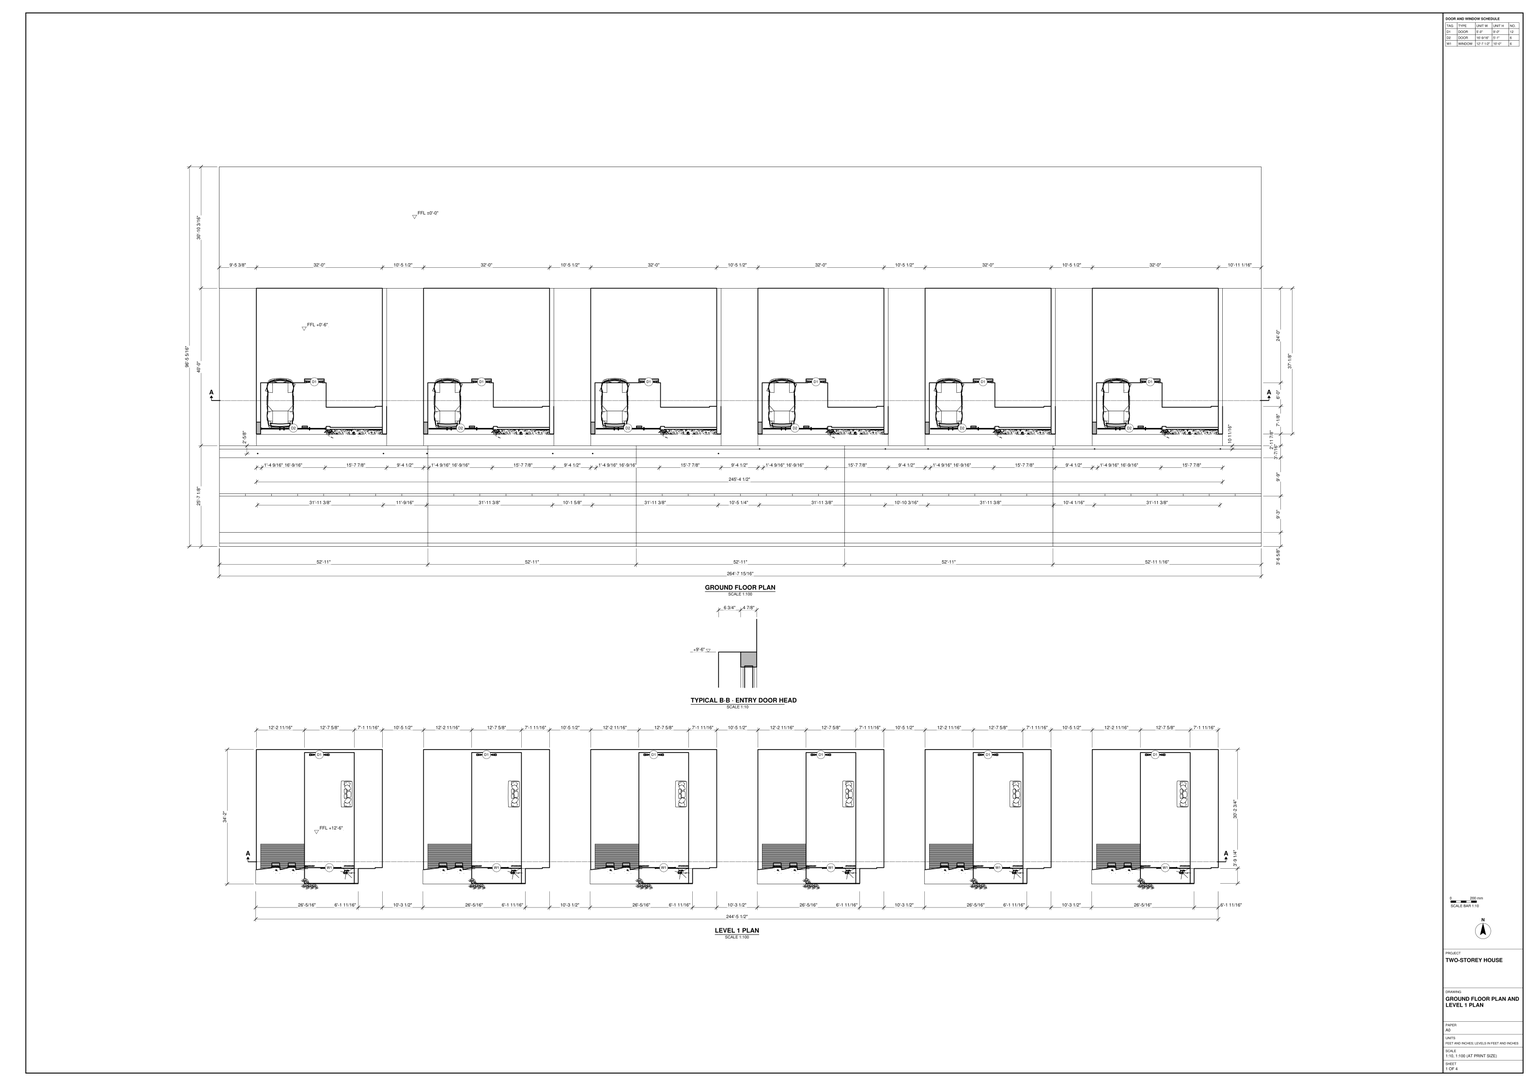
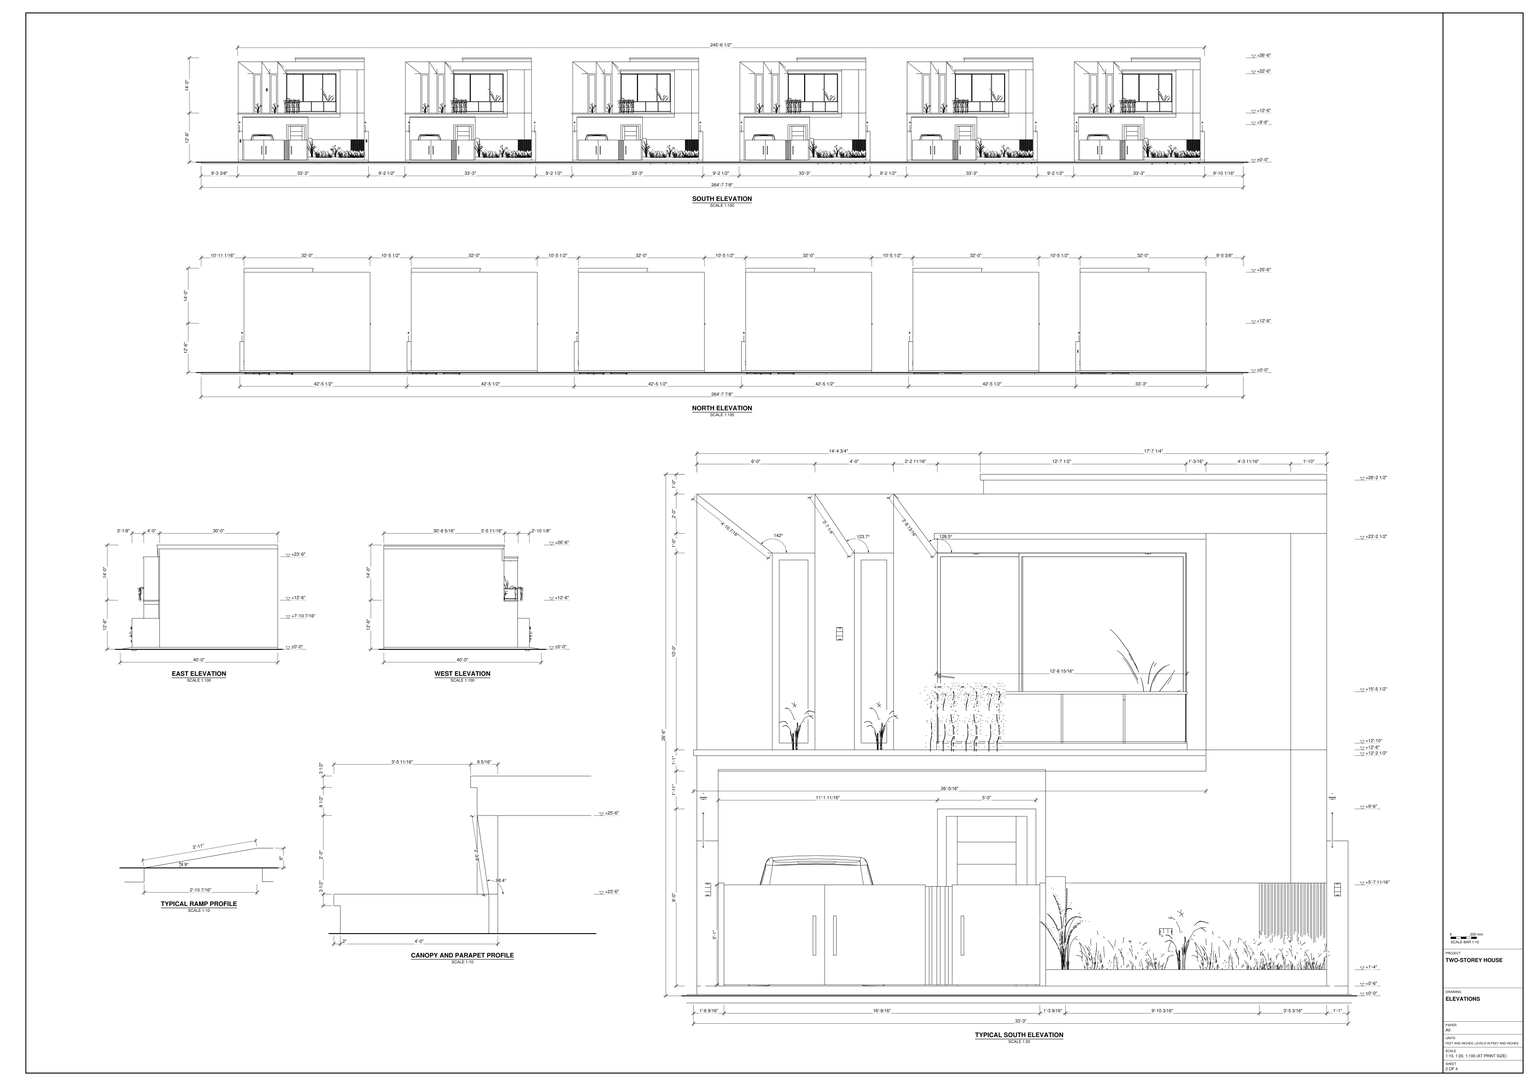
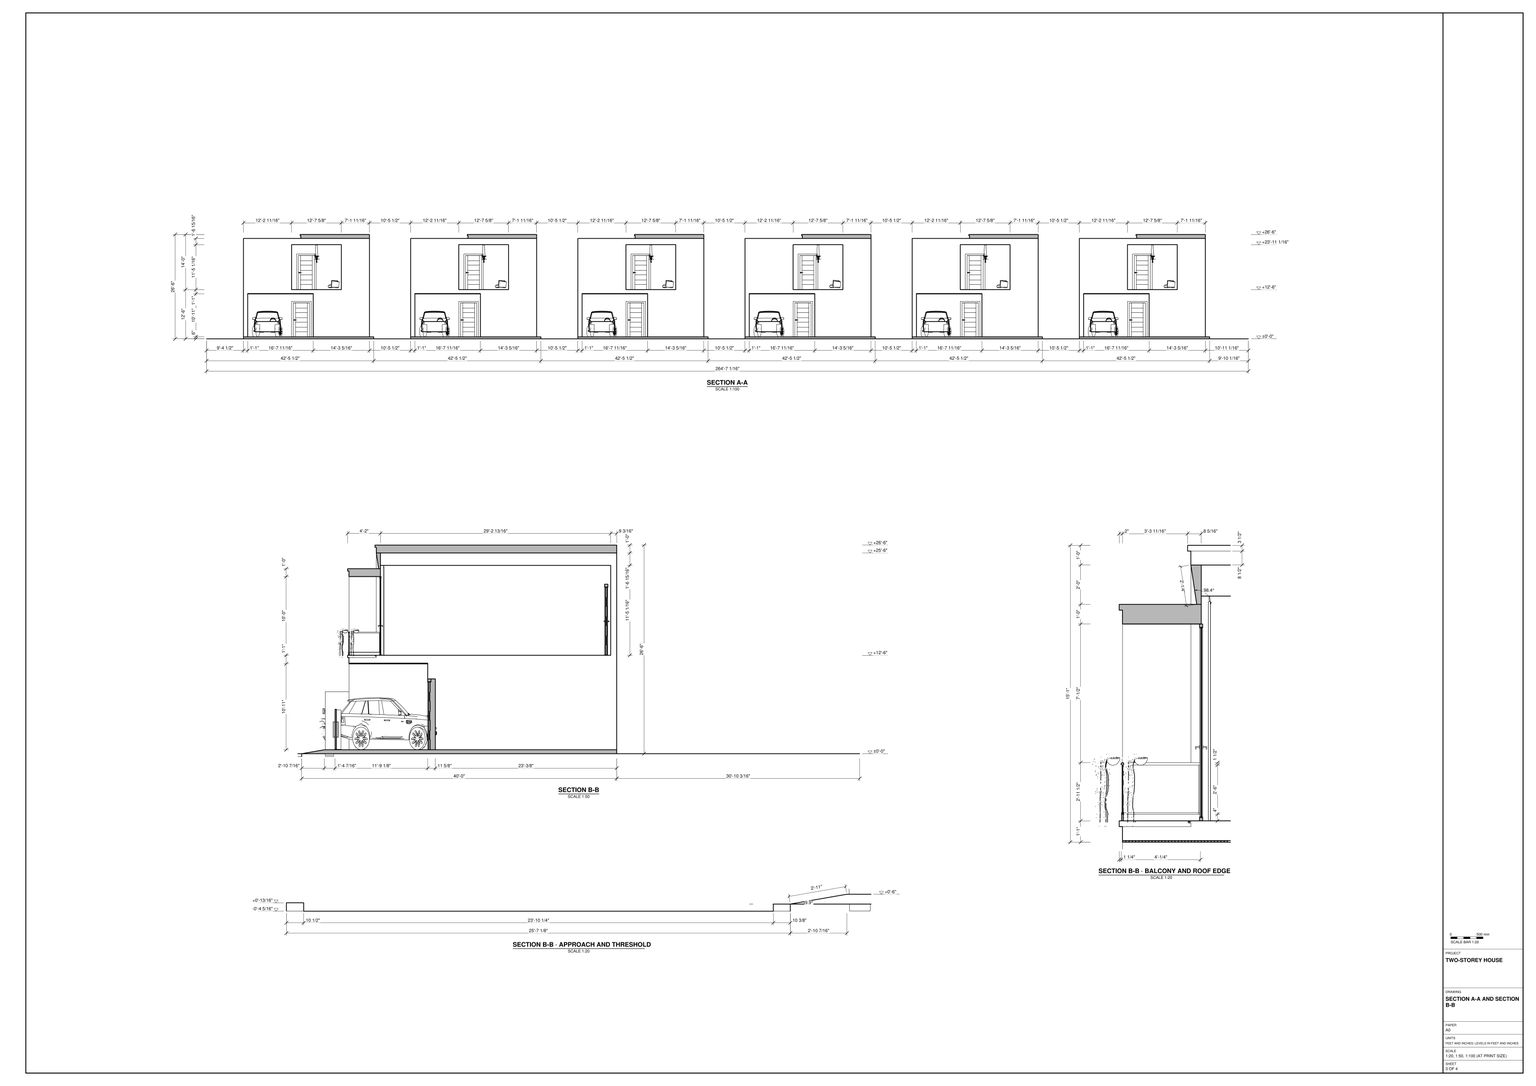
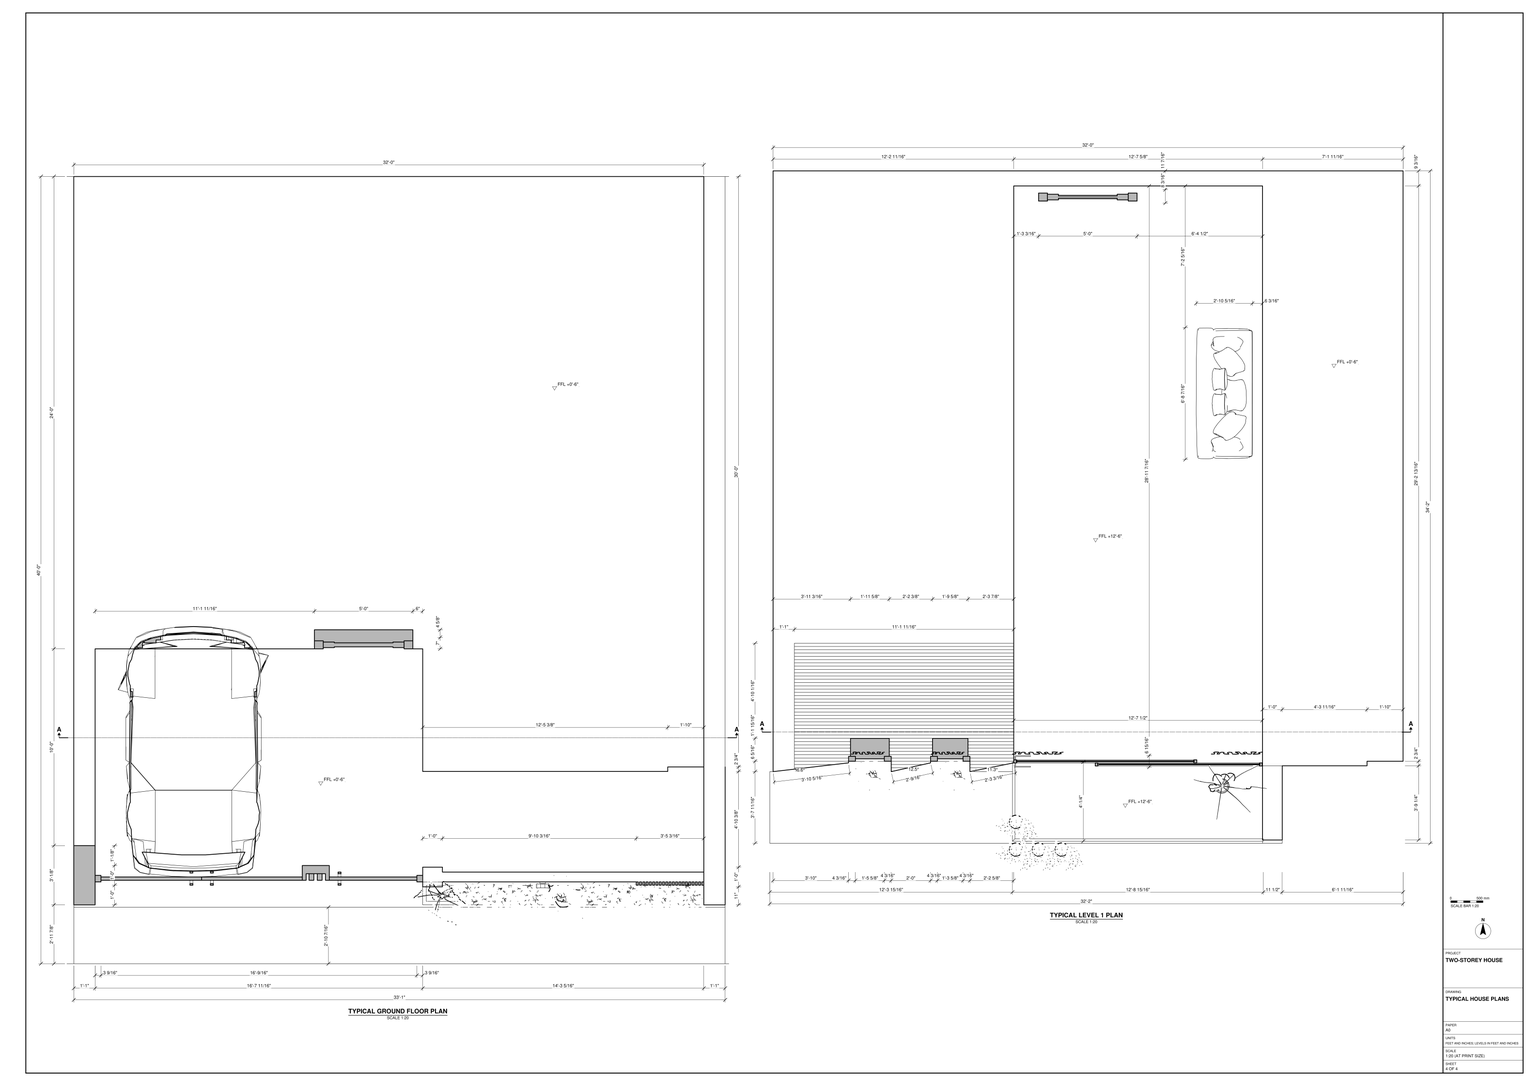
Build the six houses and their shared site in SketchUp from task_files/diagram_01.pdf. Work in feet and inches. The overall model extents are 264'-7 15/16" along the row, 96'-5 5/16" from front to back and 26'-10 5/16" in height. Set the ground-floor datum at ±0'-0" and the upper floor at +12'-6".

Use the ground-floor plan to set out the site edges, the approach across the south frontage and the gaps between houses. Model the walls at the thicknesses drawn, with floor slabs, door and window openings, flat roofs and parapets. At each frontage, form the ramped threshold, gate, covered parking bay and recessed entry. Above the bay, model the projecting balcony slab, front guard, tall fins and framed window. Use the sections to distinguish the canopy over the balcony from the higher roof edge. Include the upper-floor seating at the size and position shown in plan, together with the parked cars and planting shown in elevation. Cars, plants and other loose items may be any suitable library components.

Keep shell elements such as walls, slabs and roofs, and each furniture or joinery piece, in separate groups or components. Use components for repeated parts. Save one SketchUp model as output_files/row_of_six_two_storey_houses.skp.

# SketchUp Ruby script. Lengths in inches.
U = 1.inch
M = Sketchup.active_model
def pt(a) = Geom::Point3d.new(a.map { |v| v * U })
def face(e, loops, mat)
  f = e.add_face(loops[0].map { |a| pt(a) })
  loops[1..].each { |l| e.add_face(l.map { |a| pt(a) }).erase! }
  f.material = f.back_material = mat if mat
  f
end
# faces: each face lists its corners as indices into pts; further lists are holes
def faces(e, pts, list, mat = nil) = list.each { |f| face(e, (f[0].is_a?(Array) ? f : [f]).map { |l| l.map { |i| pts[i] } }, mat) }
# xy, xz, yz: faces in a plane at the given z, y or x. An outline is a flat list of corners, or four numbers for a rectangle; further outlines are holes
def ring(l) = l.size == 4 ? [[l[0], l[1]], [l[2], l[1]], [l[2], l[3]], [l[0], l[3]]] : l.each_slice(2).to_a
def flat(e, list, mat, &to3) = list.each { |f| face(e, (f[0].is_a?(Array) ? f : [f]).map { |l| ring(l).map { |u, v| to3.(u, v) } }, mat) }
def xy(e, z, list, mat = nil) = flat(e, list, mat) { |x, y| [x, y, z] }
def xz(e, y, list, mat = nil) = flat(e, list, mat) { |x, z| [x, y, z] }
def yz(e, x, list, mat = nil) = flat(e, list, mat) { |y, z| [x, y, z] }
def lines(e, pts, list) = list.each { |a, b| e.add_line(pt(pts[a]), pt(pts[b])) }
# prism: a flat outline (further loops are holes) pulled along v
def prism(e, loops, v, mat = nil)
  f = face(e, loops, mat); d = Geom::Vector3d.new(v.map { |x| x * U })
  f.pushpull(f.normal.samedirection?(d) ? d.length : -d.length)
end
def box(e, o, s, mat = nil) = prism(e, [[o, [o[0] + s[0], o[1], o[2]], [o[0] + s[0], o[1] + s[1], o[2]], [o[0], o[1] + s[1], o[2]]]], [0, 0, s[2]], mat)
def at(x, y, z, deg = 0) = Geom::Transformation.translation(pt([x, y, z])) * Geom::Transformation.rotation(ORIGIN, Z_AXIS, deg.degrees)
def axes(o, x, y, z) = Geom::Transformation.new([*x, 0, *y, 0, *z, 0, *pt(o).to_a, 1])
def part(name) = M.definitions.add(name)
# library, detail: a bought-in or finely detailed component or shape, given as its bounding box
def library(name, o, s) = part(name).tap { |d| box(d.entities, o, s) }
def detail(e, o, s) = box(e.add_group.entities, o, s)
def put(e, d, t, mat = nil) = e.add_instance(d, t).tap { |i| i.material = mat if mat }
def group(e, t, mat = nil) = e.add_group.tap { |g| g.transformation = t; g.material = mat if mat }.entities
root = M.entities
M.materials.add("Aluminum_Anodized_DarkGray").color = [72, 73, 74]
M.materials.add("[Asphalt_New]1").color = [67, 60, 62]
M.materials.add("[Color M09]").color = [0, 0, 0]
M.materials.add("[Color_000]").color = [255, 255, 255]
M.materials.add("[Grass Dark Green]").color = [106, 157, 55]
M.materials.add("[Pavers with Grass Brick]").color = [187, 192, 176]
M.materials.add("[Stone_Masonry_Multi]").color = [182, 175, 164]
M.materials.add("[Translucent Glass Gray]").color = [128, 128, 128]
M.materials["[Translucent Glass Gray]"].alpha = 0.5
M.materials.add("[Wood Veneer 01]").color = [120, 70, 37]
M.materials.add("polished steel").color = [183, 187, 190]
M.materials.add("polished_ Blacktop Old 01").color = [132, 136, 139]
M.materials.add("steel").color = [179, 179, 179]
c1 = library("Sliding windows",[297.42,-0.89,0.35],[192.38,8.85,122.84])
c2 = library("Pendente Fluire_RE005 ø28x74cm",[-3.08,-3.22,-55.33],[13.79,12.06,55.33])
c3 = part("faewg")
xy(c3.entities,0,[[0,-3,2,0]])
xy(c3.entities,1,[[0,-2,2,0]])
xy(c3.entities,23,[[0,-2,2,0]])
xy(c3.entities,24,[[0,-3,2,0]])
xz(c3.entities,-3,[[0,0,2,24]],"polished steel")
xz(c3.entities,-2,[[0,1,2,23]])
xz(c3.entities,0,[[0,0,2,1],[0,23,2,24]])
yz(c3.entities,0,[[-3,0,-3,24,0,24,0,23,-2,23,-2,1,0,1,0,0]])
yz(c3.entities,2,[[-3,0,0,0,0,1,-2,1,-2,23,0,23,0,24,-3,24]])
c4 = part("e3f")
xy(c4.entities,0,[[0,-2,59.93,0]])
xy(c4.entities,18,[[51.93,-5,53.93,-2]],"steel")
xy(c4.entities,19,[[51.93,-4,53.93,-2]],"steel")
xy(c4.entities,41,[[51.93,-4,53.93,-2]],"steel")
xy(c4.entities,42,[[51.93,-5,53.93,-2]],"steel")
xy(c4.entities,61,[[0,-2,59.93,0]],"[Wood Veneer 01]")
xz(c4.entities,-5,[[51.93,18,53.93,42]],"[Color M09]")
xz(c4.entities,-4,[[51.93,19,53.93,41]],"steel")
xz(c4.entities,-2,[[[0,0,59.93,61],[51.93,41,53.93,42],[51.93,18,53.93,19]]],"[Wood Veneer 01]")
xz(c4.entities,-2,[[51.93,18,53.93,19],[51.93,41,53.93,42]],"steel")
xz(c4.entities,0,[[0,0,59.93,61]],"[Wood Veneer 01]")
yz(c4.entities,0,[[-2,0,0,61]])
yz(c4.entities,51.93,[[-5,18,-5,42,-2,42,-2,41,-4,41,-4,19,-2,19,-2,18]],"[Color M09]")
yz(c4.entities,53.93,[[-5,18,-2,18,-2,19,-4,19,-4,41,-2,41,-2,42,-5,42]],"[Color M09]")
yz(c4.entities,59.93,[[-2,0,0,61]])
put(c4.entities,c3,axes([51.93,0,42],[1,0,0],[0,-1,0],[0,0,-1]),"steel")
c5 = part("reg")
xy(c5.entities,0,[[-8.95,3,59.93,5]],"[Wood Veneer 01]")
xy(c5.entities,18,[[51.93,0,53.93,3]],"[Wood Veneer 01]")
xy(c5.entities,19,[[51.93,1,53.93,3]],"[Color M09]")
xy(c5.entities,41,[[51.93,1,53.93,3]],"[Color M09]")
xy(c5.entities,42,[[51.93,0,53.93,3]],"[Color M09]")
xy(c5.entities,61,[[-8.95,3,59.93,5]],"[Wood Veneer 01]")
xz(c5.entities,0,[[51.93,18,53.93,42]],"[Color M09]")
xz(c5.entities,1,[[51.93,19,53.93,41]],"[Wood Veneer 01]")
xz(c5.entities,3,[[[-8.95,0,59.93,61],[51.93,41,53.93,42],[51.93,18,53.93,19]],[51.93,18,53.93,19],[51.93,41,53.93,42]],"[Wood Veneer 01]")
xz(c5.entities,5,[[-8.95,0,59.93,61]],"[Wood Veneer 01]")
yz(c5.entities,-8.95,[[3,0,5,61]],"[Wood Veneer 01]")
yz(c5.entities,51.93,[[0,18,0,42,3,42,3,41,1,41,1,19,3,19,3,18]],"[Color M09]")
yz(c5.entities,53.93,[[0,18,3,18,3,19,1,19,1,41,3,41,3,42,0,42]],"[Color M09]")
yz(c5.entities,59.93,[[3,0,5,61]],"[Wood Veneer 01]")
put(c5.entities,c3,axes([51.93,5.4375,42],[1,0,0],[0,-1,0],[0,0,-1]),"steel")
c6 = part("main gate")
g1 = group(c6.entities,at(416.55,56.79,1))
put(g1,c4,at(0,5,0))
put(g1,c5,axes([207.23,0,0],[-1,0,0],[0,1,0],[0,0,1]),"[Grass Dark Green]")
put(g1,c5,at(87.36,0,0),"[Grass Dark Green]")
g2 = group(g1,at(59.93,12,0),"polished_ Blacktop Old 01")
prism(g2,[[[0,0,0],[18.48,0,0],[18.48,-9,0],[15.84,-9,0],[15.84,-5,0],[2.64,-5,0],[2.64,-9,0],[0,-9,0]]],[0,0,60],"[Color M09]")
g3 = group(g1,at(-173.38,3,0),"[Grass Dark Green]")
prism(g3,[[[241.55,4,0],[241.55,4,4],[241.55,4,56],[241.55,4,60],[241.55,0,60],[241.55,0,0]]],[-3.3,0,0])
prism(g3,[[[247.19,4,0],[247.19,4,4],[247.19,4,56],[247.19,4,60],[247.19,0,60],[247.19,0,0]]],[-3.3,0,0])
c7 = library("cay+chuoi",[26.89,19.66,0.52],[41.96,45.65,69.71])
c8 = library("Areca palm plant",[0,0,0],[49.1,36.6,54.46])
c9 = library("Land Rover Range Rover Sport",[-42.64,-96.16,0],[85.02,188.78,73.23])
c10 = library("TS_VASO+GANCHOS-PARA-PENDURAR\#1",[-17.61,-15.74,-70.29],[36.55,50.24,77.96])
c11 = library("Glass Railing\#1",[-152.43,-0.75,0],[152.93,48.27,35.5])
c12 = part("Group\#12")
box(c12.entities,[0,0,0],[3.5625,4,62.75])
c13 = library("Group\#13",[0,0,0],[171.32,12,66.75])
c14 = library("door by lz",[5.91,-4.92,0],[35.43,6.61,78.47])
c15 = part("Group\#61")
p = [[0,1.89,0.38],[0,1.89,1.61],[0,0.72,0],[0,0,0.99],[0,0.72,1.99]]
lines(c15.entities,p,[[0,1],[2,0],[3,2],[4,3],[1,4]])
c16 = part("Pleated curtain panel")
p = [[20.45,2.26,80],[20.78,2.41,80]]
lines(c16.entities,p,[[0,1]])
detail(c16.entities,[0,1.93,2.7],[20.05,3.87,77.3])
put(c16.entities,c15,at(9.77,5.02,80,-180))
put(c16.entities,c15,at(11.91,5.02,80,-180))
put(c16.entities,c15,at(13.54,5.02,80,-180))
put(c16.entities,c15,at(7.29,5.02,80,-180))
put(c16.entities,c15,at(6.18,5.02,80,-180))
put(c16.entities,c15,at(8.69,5.02,80,-180))
put(c16.entities,c15,at(17.42,5.04,80,-180))
put(c16.entities,c15,at(18.86,5.04,80,-180))
put(c16.entities,c15,at(15.09,5.02,80,-180))
put(c16.entities,c15,at(16.66,5.04,80,-180))
put(c16.entities,c15,at(2.54,5.02,80,-180))
put(c16.entities,c15,at(1.38,5.02,80,-180))
put(c16.entities,c15,at(4.1,5.02,80,-180))
c17 = library("sofaD71839)",[0.35,-39.08,0.31],[80.46,34.29,30.24])
c18 = library("Group211\#1",[-99.84,-60,0],[199.68,120,1])
c19 = library("Group275\#1",[-75.83,-24,0],[151.66,48,0.08])
c20 = part("Group")
xy(c20.entities,0,[[0,-36.125,13,0],[0,0,0,408,384,408,384,48,362.03,48,362.03,45.24,212.68,45.24,212.68,120,206.68,120,206.68,131.625,146.68,131.625,146.68,120,13,120,13,0]])
xy(c20.entities,108,[[146.68,120,206.68,131.625]])
xy(c20.entities,131,[[212.68,0,310.34,45.24]])
xy(c20.entities,140.5,[[-2,-2,310.34,0],[-2,0,0,41.6875]],"Aluminum_Anodized_DarkGray")
xy(c20.entities,144,[[-2,-2,298.34,-2,298.34,398.8125,146.6875,398.8125,146.6875,41.6875,120,41.6875,120,48,96,48,96,47.02,72,41.6875,72,48,46,48,46,47.02,0,41.6875,-2,41.6875],[298.34,-2,310.34,0],[120,41.6875,146.68,41.6875,146.68,47.02],[146.68,41.6875,146.6875,41.6875,146.6875,48,146.68,47.02]])
xy(c20.entities,144,[[46,48,72,51],[96,48,120,51]],"[Color M09]")
xy(c20.entities,148.1875,[[47.1875,51,70.8125,61.9375],[97.1875,51,118.8125,61.9375]])
xy(c20.entities,148.1875,[[50.1875,48,67.8125,49.5],[100.1875,48,115.8125,49.5],[50.1875,49.5,67.8125,51],[100.1875,49.5,115.8125,51]],"[Color M09]")
xy(c20.entities,259.8125,[[50.1875,48,67.8125,49.5],[100.1875,48,115.8125,49.5],[50.1875,49.5,67.8125,51],[100.1875,49.5,115.8125,51]],"[Color M09]")
xy(c20.entities,262.8125,[[47.1875,51,70.8125,61.9375],[97.1875,51,118.8125,61.9375]])
xy(c20.entities,264,[[146.68,41.6875,146.68,47.02,146.6875,48,146.6875,41.6875],[46,47.02,72,48],[96,47.02,120,48],[146.68,47.02,146.68,48,146.6875,48]])
xy(c20.entities,264,[[46,48,72,51],[96,48,120,51]],"[Color M09]")
xy(c20.entities,272.5,[[144.68,-2,310.34,0],[144.68,0,146.68,45.24]],"Aluminum_Anodized_DarkGray")
xy(c20.entities,276,[[144.68,-2,310.34,45.24],[146.68,45.24,310.34,48],[310.34,45.24,362.03,48],[362.03,45.24,384,48]])
xy(c20.entities,281.0625,[[146.6875,48,298.34,398.8125]])
xy(c20.entities,300,[[0,41.6875,120,41.6875,120,47.02,146.68,48,384,48,384,408,0,408],[120,41.6875,146.68,48,120,47.02],[120,41.6875,384,41.6875,384,48,146.68,48]])
xz(c20.entities,-2,[[-2,140.5,310.34,144],[144.68,272.5,310.34,276]],"Aluminum_Anodized_DarkGray")
xz(c20.entities,0,[[0,0,13,88.44]])
xz(c20.entities,0,[[0,88.44,13,88.44,13,131,310.34,131,310.34,140.5,0,140.5],[298.34,144,310.34,144,310.34,272.5,146.68,272.5,146.68,264,298.34,264]],"Aluminum_Anodized_DarkGray")
xz(c20.entities,41.6875,[[-2,140.5,0,144]])
xz(c20.entities,45.24,[[212.68,0,362.03,0,362.03,144,310.34,144,310.34,131,212.68,131],[310.34,144,362.03,276],[144.68,272.5,146.68,276]])
xz(c20.entities,47.02,[[0,264,46,264,0,300],[120,264,120,300,146.68,264]])
xz(c20.entities,48,[[362.03,0,384,144],[362.03,144,384,276],[146.68,264,146.6875,276],[146.6875,264,298.34,276],[146.68,276,146.6875,300],
  [146.6875,276,298.34,281.0625],[298.34,276,384,276,384,300,146.6875,300,146.6875,281.0625,298.34,281.0625]])
xz(c20.entities,48,[[[46,144,72,264],[50.1875,148.1875,67.8125,259.8125]],[[96,144,120,264],[100.1875,148.1875,115.8125,259.8125]]],"[Color M09]")
xz(c20.entities,49.5,[[50.1875,148.1875,67.8125,259.8125],[100.1875,148.1875,115.8125,259.8125]],"[Translucent Glass Gray]")
xz(c20.entities,51,[[47.1875,148.1875,50.1875,262.8125],[67.8125,148.1875,70.8125,262.8125],[97.1875,148.1875,100.1875,262.8125],[115.8125,148.1875,118.8125,262.8125],[50.1875,259.8125,67.8125,262.8125],
  [100.1875,259.8125,115.8125,262.8125]])
xz(c20.entities,51,[[[46,144,72,264],[47.1875,148.1875,70.8125,262.8125]],[[96,144,120,264],[97.1875,148.1875,118.8125,262.8125]]],"[Color M09]")
xz(c20.entities,61.9375,[[47.1875,148.1875,70.8125,262.8125],[97.1875,148.1875,118.8125,262.8125]])
xz(c20.entities,120,[[13,0,146.68,0,146.68,108,206.68,108,206.68,0,212.68,0,212.68,131,13,131]])
xz(c20.entities,131.625,[[146.68,0,206.68,108]])
xz(c20.entities,398.8125,[[146.6875,144,298.34,281.0625]])
xz(c20.entities,408,[[0,0,384,300]])
yz(c20.entities,-2,[[-2,140.5,41.6875,144]],"Aluminum_Anodized_DarkGray")
yz(c20.entities,0,[[0,0,0,140.5,41.6875,140.5,41.6875,264,47.02,264,47.02,300,408,300,408,0],[41.6875,264,47.02,300]])
yz(c20.entities,13,[[0,0,120,131]])
yz(c20.entities,46,[[47.02,144,48,264]])
yz(c20.entities,46,[[48,144,51,264]],"[Color M09]")
yz(c20.entities,47.1875,[[51,148.1875,61.9375,262.8125]])
yz(c20.entities,50.1875,[[48,148.1875,49.5,259.8125],[49.5,148.1875,51,259.8125]],"[Color M09]")
yz(c20.entities,67.8125,[[48,148.1875,49.5,259.8125],[49.5,148.1875,51,259.8125]],"[Color M09]")
yz(c20.entities,70.8125,[[51,148.1875,61.9375,262.8125]])
yz(c20.entities,72,[[41.6875,144,41.6875,300,47.02,300,47.02,264,48,264,48,144]])
yz(c20.entities,72,[[48,144,51,264]],"[Color M09]")
yz(c20.entities,96,[[47.02,144,48,264]])
yz(c20.entities,96,[[48,144,51,264]],"[Color M09]")
yz(c20.entities,97.1875,[[51,148.1875,61.9375,262.8125]])
yz(c20.entities,100.1875,[[48,148.1875,49.5,259.8125],[49.5,148.1875,51,259.8125]],"[Color M09]")
yz(c20.entities,115.8125,[[48,148.1875,49.5,259.8125],[49.5,148.1875,51,259.8125]],"[Color M09]")
yz(c20.entities,118.8125,[[51,148.1875,61.9375,262.8125]])
yz(c20.entities,120,[[41.6875,144,41.6875,300,47.02,300,47.02,264,48,264,48,144]])
yz(c20.entities,120,[[48,144,51,264]],"[Color M09]")
yz(c20.entities,144.68,[[-2,272.5,45.24,276]],"Aluminum_Anodized_DarkGray")
yz(c20.entities,146.68,[[120,0,131.625,108],[47.02,264,45.24,276,48,276],[47.02,264,48,276,48,264]])
yz(c20.entities,146.68,[[0,264,0,272.5,45.24,272.5,45.24,276,47.02,264]],"Aluminum_Anodized_DarkGray")
yz(c20.entities,146.6875,[[48,144,398.8125,281.0625]])
yz(c20.entities,206.68,[[120,0,131.625,108]])
yz(c20.entities,212.68,[[45.24,0,120,131]])
yz(c20.entities,298.34,[[0,144,0,264,48,264,48,281.0625,398.8125,281.0625,398.8125,144]])
yz(c20.entities,310.34,[[0,131,45.24,140.5],[-2,140.5,45.24,144],[0,144,45.24,144,45.24,276,-2,276,-2,272.5,0,272.5]])
yz(c20.entities,362.03,[[45.24,0,48,144],[45.24,144,48,276]])
yz(c20.entities,384,[[48,0,408,300],[45.24,276,48,276,48,300,41.6875,300]])
p = [[46,47.02,144],[46,47.02,264],[0,41.6875,300],[0,41.6875,264],[0,41.6875,144],[96,47.02,144],
  [96,47.02,264],[72,41.6875,300],[72,41.6875,144],[146.68,47.02,144],[146.68,47.02,264],[120,41.6875,300],
  [120,41.6875,144],[146.6875,48,264],[146.6875,48,144],[72,47.02,264],[0,47.02,300],[120,47.02,264],
  [96,47.02,300],[384,41.6875,300],[146.68,45.24,276],[310.34,45.24,276],[362.03,45.24,276],[384,45.24,276],
  [146.68,48,276],[120,47.02,300],[146.68,48,300]]
faces(c20.entities,p,[[0,1,2,3,4],[5,6,7,8],[9,10,11,12],[13,10,9,14],[15,6,7,2,1],[2,16,1],[17,10,11,7,6],[18,7,6],
  [19,11,10,20,21,22,23],[10,24,11],[24,10,25],[26,11,24],[26,24,25]])
put(c20.entities,c14,axes([136.67,124.88,0],[1.69333,0,0],[0,1.24,0],[0,0,1.3764]))
put(c20.entities,c16,axes([67.8125,51.6,139.95],[-1,0,0],[0,0.36,0],[0,0,1.49853]))
put(c20.entities,c16,axes([116.4375,51.6,139.95],[-1,0,0],[0,0.36,0],[0,0,1.49853]))
put(c20.entities,c17,at(296.95,312.84,144,-90))
put(c20.entities,c14,axes([151.84,394.47,144.36],[1.69333,0,0],[0,1.24,0],[0,0,1.3764]))
put(c20.entities,c16,axes([176.8125,51.6,139.33],[-1.54082,0,0],[0,0.36,0],[0,0,1.7287]))
put(c20.entities,c16,axes([298,51.6,139.33],[-1.54082,0,0],[0,0.36,0],[0,0,1.7287]))
g4 = group(c20.entities,at(0,-36.125,0))
xy(g4,88.44,[[0,0,13,36.125]])
xz(g4,0,[[0,0,13,88.44]])
yz(g4,0,[[0,0,36.125,88.44]])
yz(g4,13,[[0,0,36.125,88.44]])
g5 = group(c20.entities,at(384,11.875,0))
xy(g5,88.44,[[0,-48,13,36.125]])
xz(g5,-48,[[0,0,13,88.44]])
yz(g5,0,[[-48,0,36.125,88.44]])
yz(g5,13,[[-48,0,36.125,88.44]])
put(c20.entities,c18,at(112.84,60,131),"[Wood Veneer 01]")
put(c20.entities,c19,at(222.51,24,264),"[Wood Veneer 01]")
c21 = part("Group\#1")
xy(c21.entities,0,[[48,0,445,480]])
xy(c21.entities,6,[[48,34.46,445,480]])
xz(c21.entities,480,[[48,0,445,6]])
yz(c21.entities,48,[[0,0,34.46,6,480,6,480,0]])
yz(c21.entities,445,[[0,0,480,0,480,6,34.46,6]])
p = [[445,0,0],[445,34.46,6],[48,34.46,6],[48,0,0]]
faces(c21.entities,p,[[0,1,2,3]],"[Pavers with Grass Brick]")
c22 = library("Group20\#2",[-20.81,-17.08,3.79],[39.86,39.43,37.51])
c23 = part("Group\#14")
xy(c23.entities,0,[[0,0,171.32,14]])
xy(c23.entities,6.8125,[[2.1875,2.1875,169.14,11.8125]])
xy(c23.entities,10,[[[0,0,171.32,14],[2.1875,2.1875,169.14,11.8125]]])
xz(c23.entities,0,[[0,0,171.32,10]])
xz(c23.entities,2.1875,[[2.1875,6.8125,169.14,10]])
xz(c23.entities,11.8125,[[2.1875,6.8125,169.14,10]])
xz(c23.entities,14,[[0,0,171.32,10]])
yz(c23.entities,0,[[0,0,14,10]])
yz(c23.entities,2.1875,[[2.1875,6.8125,11.8125,10]])
yz(c23.entities,169.14,[[2.1875,6.8125,11.8125,10]])
yz(c23.entities,171.32,[[0,0,14,10]])
c24 = library("Group8\#2",[-183.25,9.15,0],[25.91,56.79,43.93])
c25 = part("Two-storey house")
xy(c25.entities,4.1875,[[0,0,112.5,480]],"[Grass Dark Green]")
put(c25.entities,c1,axes([24.94,117.14,153.87],[0.7875,0,0],[0,0.7875,0],[0,0,0.97692]))
put(c25.entities,c2,at(332.14,291.17,291.84))
put(c25.entities,c6,axes([692.63,-8.92,9.89],[-0.89069,0,0],[0,1,0],[0,0,1]))
put(c25.entities,c7,at(395.27,42.99,157.67,55))
put(c25.entities,c8,axes([335.92,13.95,16.21],[0.56191,0.45017,0],[-0.65172,0.81348,0],[0,0,1.1151]))
put(c25.entities,c9,axes([185.49,127.89,10.1875],[1.09,0,0],[0,-0.80991,0],[0,0,1.08608]))
put(c25.entities,c10,axes([255.57,79.83,191.71],[0.12065,0.57753,0],[0.57753,-0.12065,0],[0,0,0.59]))
put(c25.entities,c10,axes([269.51,62.95,191.71],[0.12065,0.57753,0],[0.57753,-0.12065,0],[0,0,0.59]))
put(c25.entities,c10,axes([283.45,62.95,191.71],[0.12065,0.57753,0],[0.57753,-0.12065,0],[0,0,0.59]))
put(c25.entities,c10,axes([255.57,62.95,191.71],[0.12065,0.57753,0],[0.57753,-0.12065,0],[0,0,0.59]))
put(c25.entities,c11,at(410.84,72,154.1875))
g6 = group(c25.entities,at(339.875,113.6875,310.1875),"Aluminum_Anodized_DarkGray")
xy(g6,0,[[-52.625,0,156.625,366.3125]])
xy(g6,8.5,[[-54.625,-2,156.625,0],[-54.625,0,-52.625,366.3125]])
xy(g6,12,[[-54.625,-2,156.625,366.3125]],"Aluminum_Anodized_DarkGray")
xz(g6,-2,[[-54.625,8.5,156.625,12]],"Aluminum_Anodized_DarkGray")
xz(g6,0,[[-52.625,0,156.625,8.5]],"Aluminum_Anodized_DarkGray")
xz(g6,366.3125,[[-52.625,0,-52.625,8.5,-54.625,8.5,-54.625,12,156.625,12,156.625,0]])
yz(g6,-54.625,[[-2,8.5,366.3125,12]],"Aluminum_Anodized_DarkGray")
yz(g6,-52.625,[[0,0,366.3125,8.5]],"Aluminum_Anodized_DarkGray")
yz(g6,156.625,[[0,0,366.3125,0,366.3125,12,-2,12,-2,8.5,0,8.5]])
put(c25.entities,c12,at(321.61,49.87,10.1875),"[Color M09]")
put(c25.entities,c13,at(325.18,46.875,10.1875))
put(c25.entities,c20,at(112.5,72,10.1875))
put(c25.entities,c21,at(64.5,0,4.1875))
put(c25.entities,c22,axes([173.64,113.8,149.34],[-0.76108,0,0],[0,-0.646,0],[0,0,0.85272]))
put(c25.entities,c22,axes([225.2,113.8,149.34],[-0.76108,0,0],[0,-0.646,0],[0,0,0.85272]))
put(c25.entities,c22,axes([409.8125,42.27,12.0625],[-1.00142,0,0],[0,-0.85,0],[0,0,1.122]))
put(c25.entities,c23,at(325.18,35.875,10.1875))
put(c25.entities,c24,axes([332.55,-127.87,0],[0,-1,0],[1.09,0,0],[0,0,1]))
put(c25.entities,c24,axes([403.03,-127.87,0],[0,-1,0],[1.08,0,0],[0,0,1]))
put(c25.entities,c24,at(433.63,-127.87,0,-90))
c26 = part("weg 1")
xy(c26.entities,0,[[119.79,-0.03,149.12,635.01],[405.36,-0.03,441.44,635.01]])
xy(c26.entities,0,[[149.12,-0.03,272.68,635.01],[272.68,-0.03,280.61,79.35],[280.61,-0.03,405.36,635.01],[272.68,158.73,280.61,238.11],[272.68,317.49,280.61,396.87],
  [272.68,476.25,280.61,555.63]],"[Asphalt_New]1")
xy(c26.entities,0,[[272.68,79.35,280.61,158.73],[272.68,238.11,280.61,317.49],[272.68,396.87,280.61,476.25],[272.68,555.63,280.61,635.01]],"[Color_000]")
xy(c26.entities,4.33,[[108.17,0,119.79,635.01]],"[Stone_Masonry_Multi]")
xy(c26.entities,5.12,[[441.44,-0.03,453.25,635.01]],"[Stone_Masonry_Multi]")
xz(c26.entities,-0.03,[[441.44,0,453.25,5.12]],"[Stone_Masonry_Multi]")
xz(c26.entities,0,[[108.17,0,119.79,4.33]],"[Stone_Masonry_Multi]")
xz(c26.entities,635.01,[[108.17,0,119.79,4.33],[441.44,0,453.25,5.12]],"[Stone_Masonry_Multi]")
yz(c26.entities,108.17,[[0,0,635.01,4.33]],"[Stone_Masonry_Multi]")
yz(c26.entities,119.79,[[0,0,635.01,4.33]],"[Stone_Masonry_Multi]")
yz(c26.entities,441.44,[[-0.03,0,635.01,5.12]],"[Stone_Masonry_Multi]")
yz(c26.entities,453.25,[[-0.03,0,635.01,5.12]],"[Stone_Masonry_Multi]")
c27 = library("[SKP_VZ_MOD_01]_WALL_LIGHT",[-1.37,-1.22,0],[3.81,2.36,6.3])
c28 = library("IES Light\#1",[-4.45,-4.45,-12],[8.9,8.9,12])
c29 = library("IES Light\#2",[-4.45,-4.45,-12],[8.9,8.9,12])
c30 = library("Group\#44",[0,0,0],[4.9,41.21,123.37])
c31 = library("Group\#54",[0,0,0.375],[3.5,3.5,0.5625])
xy(root,0,[[0,787.12,3175.9375,1157.31]],"[Grass Dark Green]")
put(root,c25,at(0.89,307.12,-4.1875))
put(root,c26,axes([0.89,403.39,-4.33],[0,-0.89,0],[1,0,0],[0,0,1]))
put(root,c26,axes([635.9,403.39,-4.33],[0,-0.89,0],[1,0,0],[0,0,1]))
put(root,c26,axes([1270.91,403.39,-4.33],[0,-0.89,0],[1,0,0],[0,0,1]))
put(root,c26,axes([1905.92,403.39,-4.33],[0,-0.89,0],[1,0,0],[0,0,1]))
put(root,c26,axes([2540.93,403.39,-4.33],[0,-0.89,0],[1,0,0],[0,0,1]))
put(root,c27,at(118.47,433.43,64.45,90))
put(root,c27,axes([119.86,340.56,60.88],[0,1,0],[-1.66,0,0],[0,0,1.25]))
put(root,c27,axes([503.86,340.56,60.88],[0,1,0],[-1.66,0,0],[0,0,1.25]))
put(root,c27,axes([200.4,421.74,216.86],[-0.17021,0.98541,0],[-1.63578,-0.28255,0],[0,0,1.25]))
put(root,c27,axes([395.3,354.42,39.18],[0,1,0],[0,0,1.66],[1.25,0,0]))
put(root,c28,at(283.61,400.18,269.05))
put(root,c28,at(388.27,400.18,269.05))
put(root,c29,at(117.44,257.98,119.65))
put(root,c12,at(126.39,357,6),"[Color M09]")
g7 = group(root,at(510.39,307.12,-4.1875))
xy(g7,4.1875,[[0,0,112.5,480]],"[Grass Dark Green]")
put(g7,c1,axes([24.94,117.14,153.87],[0.7875,0,0],[0,0.7875,0],[0,0,0.97692]))
put(g7,c2,at(332.14,291.17,291.84))
put(g7,c6,axes([692.63,-8.92,9.89],[-0.89069,0,0],[0,1,0],[0,0,1]))
put(g7,c7,at(395.27,42.99,157.67,55))
put(g7,c8,axes([335.92,13.95,16.21],[0.56191,0.45017,0],[-0.65172,0.81348,0],[0,0,1.1151]))
put(g7,c9,axes([185.49,127.89,10.1875],[1.09,0,0],[0,-0.80991,0],[0,0,1.08608]))
put(g7,c10,axes([255.57,79.83,191.71],[0.12065,0.57753,0],[0.57753,-0.12065,0],[0,0,0.59]))
put(g7,c10,axes([269.51,62.95,191.71],[0.12065,0.57753,0],[0.57753,-0.12065,0],[0,0,0.59]))
put(g7,c10,axes([283.45,62.95,191.71],[0.12065,0.57753,0],[0.57753,-0.12065,0],[0,0,0.59]))
put(g7,c10,axes([255.57,62.95,191.71],[0.12065,0.57753,0],[0.57753,-0.12065,0],[0,0,0.59]))
put(g7,c11,at(410.84,72,154.1875))
g8 = group(g7,at(339.875,113.6875,310.1875))
xy(g8,0,[[-52.625,0,156.625,366.3125]])
xy(g8,8.5,[[-54.625,-2,156.625,0],[-54.625,0,-52.625,366.3125]])
xy(g8,12,[[-54.625,-2,156.625,366.3125]],"Aluminum_Anodized_DarkGray")
xz(g8,-2,[[-54.625,8.5,156.625,12]],"Aluminum_Anodized_DarkGray")
xz(g8,0,[[-52.625,0,156.625,8.5]],"Aluminum_Anodized_DarkGray")
xz(g8,366.3125,[[-52.625,0,-52.625,8.5,-54.625,8.5,-54.625,12,156.625,12,156.625,0]])
yz(g8,-54.625,[[-2,8.5,366.3125,12]],"Aluminum_Anodized_DarkGray")
yz(g8,-52.625,[[0,0,366.3125,8.5]],"Aluminum_Anodized_DarkGray")
yz(g8,156.625,[[0,0,366.3125,0,366.3125,12,-2,12,-2,8.5,0,8.5]],"Aluminum_Anodized_DarkGray")
put(g7,c12,at(321.61,49.87,10.1875),"[Color M09]")
put(g7,c13,at(325.18,46.875,10.1875))
put(g7,c20,at(112.5,72,10.1875))
put(g7,c21,at(64.5,0,4.1875))
put(g7,c22,axes([173.64,113.8,149.34],[-0.76108,0,0],[0,-0.646,0],[0,0,0.85272]))
put(g7,c22,axes([225.2,113.8,149.34],[-0.76108,0,0],[0,-0.646,0],[0,0,0.85272]))
put(g7,c22,axes([409.8125,42.27,12.0625],[-1.00142,0,0],[0,-0.85,0],[0,0,1.122]))
put(g7,c23,at(325.18,35.875,10.1875))
put(g7,c24,axes([332.55,-127.87,0],[0,-1,0],[1.09,0,0],[0,0,1]))
put(g7,c24,axes([403.03,-127.87,0],[0,-1,0],[1.08,0,0],[0,0,1]))
put(g7,c24,at(433.63,-127.87,0,-90))
g9 = group(root,at(1019.89,307.12,-4.1875))
xy(g9,4.1875,[[0,0,112.5,480]],"[Grass Dark Green]")
put(g9,c1,axes([24.94,117.14,153.87],[0.7875,0,0],[0,0.7875,0],[0,0,0.97692]))
put(g9,c2,at(332.14,291.17,291.84))
put(g9,c6,axes([692.63,-8.92,9.89],[-0.89069,0,0],[0,1,0],[0,0,1]))
put(g9,c7,at(395.27,42.99,157.67,55))
put(g9,c8,axes([335.92,13.95,16.21],[0.56191,0.45017,0],[-0.65172,0.81348,0],[0,0,1.1151]))
put(g9,c9,axes([185.49,127.89,10.1875],[1.09,0,0],[0,-0.80991,0],[0,0,1.08608]))
put(g9,c10,axes([255.57,79.83,191.71],[0.12065,0.57753,0],[0.57753,-0.12065,0],[0,0,0.59]))
put(g9,c10,axes([269.51,62.95,191.71],[0.12065,0.57753,0],[0.57753,-0.12065,0],[0,0,0.59]))
put(g9,c10,axes([283.45,62.95,191.71],[0.12065,0.57753,0],[0.57753,-0.12065,0],[0,0,0.59]))
put(g9,c10,axes([255.57,62.95,191.71],[0.12065,0.57753,0],[0.57753,-0.12065,0],[0,0,0.59]))
put(g9,c11,at(410.84,72,154.1875))
g10 = group(g9,at(339.875,113.6875,310.1875))
xy(g10,0,[[-52.625,0,156.625,366.3125]])
xy(g10,8.5,[[-54.625,-2,156.625,0],[-54.625,0,-52.625,366.3125]])
xy(g10,12,[[-54.625,-2,156.625,366.3125]],"Aluminum_Anodized_DarkGray")
xz(g10,-2,[[-54.625,8.5,156.625,12]],"Aluminum_Anodized_DarkGray")
xz(g10,0,[[-52.625,0,156.625,8.5]],"Aluminum_Anodized_DarkGray")
xz(g10,366.3125,[[-52.625,0,-52.625,8.5,-54.625,8.5,-54.625,12,156.625,12,156.625,0]])
yz(g10,-54.625,[[-2,8.5,366.3125,12]],"Aluminum_Anodized_DarkGray")
yz(g10,-52.625,[[0,0,366.3125,8.5]],"Aluminum_Anodized_DarkGray")
yz(g10,156.625,[[0,0,366.3125,0,366.3125,12,-2,12,-2,8.5,0,8.5]],"Aluminum_Anodized_DarkGray")
put(g9,c12,at(321.61,49.87,10.1875),"[Color M09]")
put(g9,c13,at(325.18,46.875,10.1875))
put(g9,c20,at(112.5,72,10.1875))
put(g9,c21,at(64.5,0,4.1875))
put(g9,c22,axes([173.64,113.8,149.34],[-0.76108,0,0],[0,-0.646,0],[0,0,0.85272]))
put(g9,c22,axes([225.2,113.8,149.34],[-0.76108,0,0],[0,-0.646,0],[0,0,0.85272]))
put(g9,c22,axes([409.8125,42.27,12.0625],[-1.00142,0,0],[0,-0.85,0],[0,0,1.122]))
put(g9,c23,at(325.18,35.875,10.1875))
put(g9,c24,axes([332.55,-127.87,0],[0,-1,0],[1.09,0,0],[0,0,1]))
put(g9,c24,axes([403.03,-127.87,0],[0,-1,0],[1.08,0,0],[0,0,1]))
put(g9,c24,at(433.63,-127.87,0,-90))
g11 = group(root,at(1529.39,307.12,-4.1875))
xy(g11,4.1875,[[0,0,112.5,480]],"[Grass Dark Green]")
put(g11,c1,axes([24.94,117.14,153.87],[0.7875,0,0],[0,0.7875,0],[0,0,0.97692]))
put(g11,c2,at(332.14,291.17,291.84))
put(g11,c6,axes([692.63,-8.92,9.89],[-0.89069,0,0],[0,1,0],[0,0,1]))
put(g11,c7,at(395.27,42.99,157.67,55))
put(g11,c8,axes([335.92,13.95,16.21],[0.56191,0.45017,0],[-0.65172,0.81348,0],[0,0,1.1151]))
put(g11,c9,axes([185.49,127.89,10.1875],[1.09,0,0],[0,-0.80991,0],[0,0,1.08608]))
put(g11,c10,axes([255.57,79.83,191.71],[0.12065,0.57753,0],[0.57753,-0.12065,0],[0,0,0.59]))
put(g11,c10,axes([269.51,62.95,191.71],[0.12065,0.57753,0],[0.57753,-0.12065,0],[0,0,0.59]))
put(g11,c10,axes([283.45,62.95,191.71],[0.12065,0.57753,0],[0.57753,-0.12065,0],[0,0,0.59]))
put(g11,c10,axes([255.57,62.95,191.71],[0.12065,0.57753,0],[0.57753,-0.12065,0],[0,0,0.59]))
put(g11,c11,at(410.84,72,154.1875))
g12 = group(g11,at(339.875,113.6875,310.1875))
xy(g12,0,[[-52.625,0,156.625,366.3125]])
xy(g12,8.5,[[-54.625,-2,156.625,0],[-54.625,0,-52.625,366.3125]])
xy(g12,12,[[-54.625,-2,156.625,366.3125]],"Aluminum_Anodized_DarkGray")
xz(g12,-2,[[-54.625,8.5,156.625,12]],"Aluminum_Anodized_DarkGray")
xz(g12,0,[[-52.625,0,156.625,8.5]],"Aluminum_Anodized_DarkGray")
xz(g12,366.3125,[[-52.625,0,-52.625,8.5,-54.625,8.5,-54.625,12,156.625,12,156.625,0]])
yz(g12,-54.625,[[-2,8.5,366.3125,12]],"Aluminum_Anodized_DarkGray")
yz(g12,-52.625,[[0,0,366.3125,8.5]],"Aluminum_Anodized_DarkGray")
yz(g12,156.625,[[0,0,366.3125,0,366.3125,12,-2,12,-2,8.5,0,8.5]])
put(g11,c12,at(321.61,49.87,10.1875),"[Color M09]")
put(g11,c13,at(325.18,46.875,10.1875))
put(g11,c20,at(112.5,72,10.1875))
put(g11,c21,at(64.5,0,4.1875))
put(g11,c22,axes([173.64,113.8,149.34],[-0.76108,0,0],[0,-0.646,0],[0,0,0.85272]))
put(g11,c22,axes([225.2,113.8,149.34],[-0.76108,0,0],[0,-0.646,0],[0,0,0.85272]))
put(g11,c22,axes([409.8125,42.27,12.0625],[-1.00142,0,0],[0,-0.85,0],[0,0,1.122]))
put(g11,c23,at(325.18,35.875,10.1875))
put(g11,c24,axes([332.55,-127.87,0],[0,-1,0],[1.09,0,0],[0,0,1]))
put(g11,c24,axes([403.03,-127.87,0],[0,-1,0],[1.08,0,0],[0,0,1]))
put(g11,c24,at(433.63,-127.87,0,-90))
g13 = group(root,at(2038.89,307.12,-4.1875))
xy(g13,4.1875,[[0,0,112.5,480]],"[Grass Dark Green]")
put(g13,c1,axes([24.94,117.14,153.87],[0.7875,0,0],[0,0.7875,0],[0,0,0.97692]))
put(g13,c2,at(332.14,291.17,291.84))
put(g13,c6,axes([692.63,-8.92,9.89],[-0.89069,0,0],[0,1,0],[0,0,1]))
put(g13,c7,at(395.27,42.99,157.67,55))
put(g13,c8,axes([335.92,13.95,16.21],[0.56191,0.45017,0],[-0.65172,0.81348,0],[0,0,1.1151]))
put(g13,c9,axes([185.49,127.89,10.1875],[1.09,0,0],[0,-0.80991,0],[0,0,1.08608]))
put(g13,c10,axes([255.57,79.83,191.71],[0.12065,0.57753,0],[0.57753,-0.12065,0],[0,0,0.59]))
put(g13,c10,axes([269.51,62.95,191.71],[0.12065,0.57753,0],[0.57753,-0.12065,0],[0,0,0.59]))
put(g13,c10,axes([283.45,62.95,191.71],[0.12065,0.57753,0],[0.57753,-0.12065,0],[0,0,0.59]))
put(g13,c10,axes([255.57,62.95,191.71],[0.12065,0.57753,0],[0.57753,-0.12065,0],[0,0,0.59]))
put(g13,c11,at(410.84,72,154.1875))
g14 = group(g13,at(339.875,113.6875,310.1875))
xy(g14,0,[[-52.625,0,156.625,366.3125]])
xy(g14,8.5,[[-54.625,-2,156.625,0],[-54.625,0,-52.625,366.3125]])
xy(g14,12,[[-54.625,-2,156.625,366.3125]],"Aluminum_Anodized_DarkGray")
xz(g14,-2,[[-54.625,8.5,156.625,12]],"Aluminum_Anodized_DarkGray")
xz(g14,0,[[-52.625,0,156.625,8.5]],"Aluminum_Anodized_DarkGray")
xz(g14,366.3125,[[-52.625,0,-52.625,8.5,-54.625,8.5,-54.625,12,156.625,12,156.625,0]])
yz(g14,-54.625,[[-2,8.5,366.3125,12]],"Aluminum_Anodized_DarkGray")
yz(g14,-52.625,[[0,0,366.3125,8.5]],"Aluminum_Anodized_DarkGray")
yz(g14,156.625,[[0,0,366.3125,0,366.3125,12,-2,12,-2,8.5,0,8.5]])
put(g13,c12,at(321.61,49.87,10.1875),"[Color M09]")
put(g13,c13,at(325.18,46.875,10.1875))
put(g13,c20,at(112.5,72,10.1875))
put(g13,c21,at(64.5,0,4.1875))
put(g13,c22,axes([173.64,113.8,149.34],[-0.76108,0,0],[0,-0.646,0],[0,0,0.85272]))
put(g13,c22,axes([225.2,113.8,149.34],[-0.76108,0,0],[0,-0.646,0],[0,0,0.85272]))
put(g13,c22,axes([409.8125,42.27,12.0625],[-1.00142,0,0],[0,-0.85,0],[0,0,1.122]))
put(g13,c23,at(325.18,35.875,10.1875))
put(g13,c24,axes([332.55,-127.87,0],[0,-1,0],[1.09,0,0],[0,0,1]))
put(g13,c24,axes([403.03,-127.87,0],[0,-1,0],[1.08,0,0],[0,0,1]))
put(g13,c24,at(433.63,-127.87,0,-90))
g15 = group(root,at(2548.39,307.12,-4.1875))
xy(g15,4.1875,[[0,0,112.5,480],[509.5,0,627.55,480]],"[Grass Dark Green]")
put(g15,c1,axes([24.94,117.14,153.87],[0.7875,0,0],[0,0.7875,0],[0,0,0.97692]))
put(g15,c2,at(332.14,291.17,291.84))
put(g15,c6,axes([692.63,-8.92,9.89],[-0.89069,0,0],[0,1,0],[0,0,1]))
put(g15,c7,at(395.27,42.99,157.67,55))
put(g15,c8,axes([335.92,13.95,16.21],[0.56191,0.45017,0],[-0.65172,0.81348,0],[0,0,1.1151]))
put(g15,c9,axes([185.49,127.89,10.1875],[1.09,0,0],[0,-0.80991,0],[0,0,1.08608]))
put(g15,c10,axes([255.57,79.83,191.71],[0.12065,0.57753,0],[0.57753,-0.12065,0],[0,0,0.59]))
put(g15,c10,axes([269.51,62.95,191.71],[0.12065,0.57753,0],[0.57753,-0.12065,0],[0,0,0.59]))
put(g15,c10,axes([283.45,62.95,191.71],[0.12065,0.57753,0],[0.57753,-0.12065,0],[0,0,0.59]))
put(g15,c10,axes([255.57,62.95,191.71],[0.12065,0.57753,0],[0.57753,-0.12065,0],[0,0,0.59]))
put(g15,c11,at(410.84,72,154.1875))
g16 = group(g15,at(339.875,113.6875,310.1875))
xy(g16,0,[[-52.625,0,156.625,366.3125]])
xy(g16,8.5,[[-54.625,-2,156.625,0],[-54.625,0,-52.625,366.3125]])
xy(g16,12,[[-54.625,-2,156.625,366.3125]],"Aluminum_Anodized_DarkGray")
xz(g16,-2,[[-54.625,8.5,156.625,12]],"Aluminum_Anodized_DarkGray")
xz(g16,0,[[-52.625,0,156.625,8.5]],"Aluminum_Anodized_DarkGray")
xz(g16,366.3125,[[-52.625,0,-52.625,8.5,-54.625,8.5,-54.625,12,156.625,12,156.625,0]])
yz(g16,-54.625,[[-2,8.5,366.3125,12]],"Aluminum_Anodized_DarkGray")
yz(g16,-52.625,[[0,0,366.3125,8.5]],"Aluminum_Anodized_DarkGray")
yz(g16,156.625,[[0,0,366.3125,0,366.3125,12,-2,12,-2,8.5,0,8.5]])
put(g15,c12,at(321.61,49.87,10.1875),"[Color M09]")
put(g15,c13,at(325.18,46.875,10.1875))
put(g15,c20,at(112.5,72,10.1875))
put(g15,c21,at(64.5,0,4.1875))
put(g15,c22,axes([173.64,113.8,149.34],[-0.76108,0,0],[0,-0.646,0],[0,0,0.85272]))
put(g15,c22,axes([225.2,113.8,149.34],[-0.76108,0,0],[0,-0.646,0],[0,0,0.85272]))
put(g15,c22,axes([409.8125,42.27,12.0625],[-1.00142,0,0],[0,-0.85,0],[0,0,1.122]))
put(g15,c23,at(325.18,35.875,10.1875))
put(g15,c24,axes([332.55,-127.87,0],[0,-1,0],[1.09,0,0],[0,0,1]))
put(g15,c24,axes([403.03,-127.87,0],[0,-1,0],[1.08,0,0],[0,0,1]))
put(g15,c24,at(433.63,-127.87,0,-90))
put(root,c30,axes([114.9,255.125,0],[1,0,0],[0,0.71,0],[0,0,1]))
put(root,c30,axes([498.27,255.125,0],[1,0,0],[0,0.71,0],[0,0,1]))
put(root,c30,axes([630.87,255.125,0],[1,0,0],[0,0.71,0],[0,0,1]))
put(root,c30,axes([1014.24,255.125,0],[1,0,0],[0,0.71,0],[0,0,1]))
put(root,c30,axes([1519.24,255.125,0],[1,0,0],[0,0.71,0],[0,0,1]))
put(root,c30,axes([1135.87,255.125,0],[1,0,0],[0,0.71,0],[0,0,1]))
put(root,c30,axes([2027.89,269.07,0],[1,0,0],[0,0.71,0],[0,0,1]))
put(root,c30,axes([1644.51,269.07,0],[1,0,0],[0,0.71,0],[0,0,1]))
put(root,c30,axes([2158.07,269.07,0],[1,0,0],[0,0.71,0],[0,0,1]))
put(root,c30,axes([2541.45,269.07,0],[1,0,0],[0,0.71,0],[0,0,1]))
put(root,c30,axes([2665.51,269.07,0],[1,0,0],[0,0.71,0],[0,0,1]))
put(root,c30,axes([3048.89,269.07,0],[1,0,0],[0,0.71,0],[0,0,1]))
put(root,c31,at(281.86,398.43,269.0625))
put(root,c31,at(386.61,398.43,269.0625))
